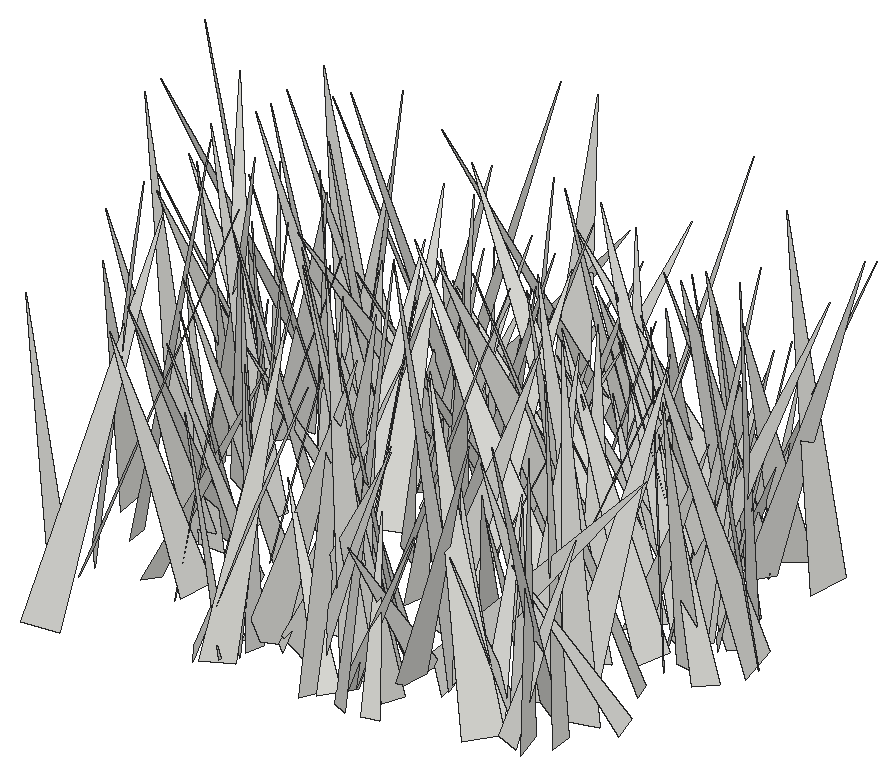
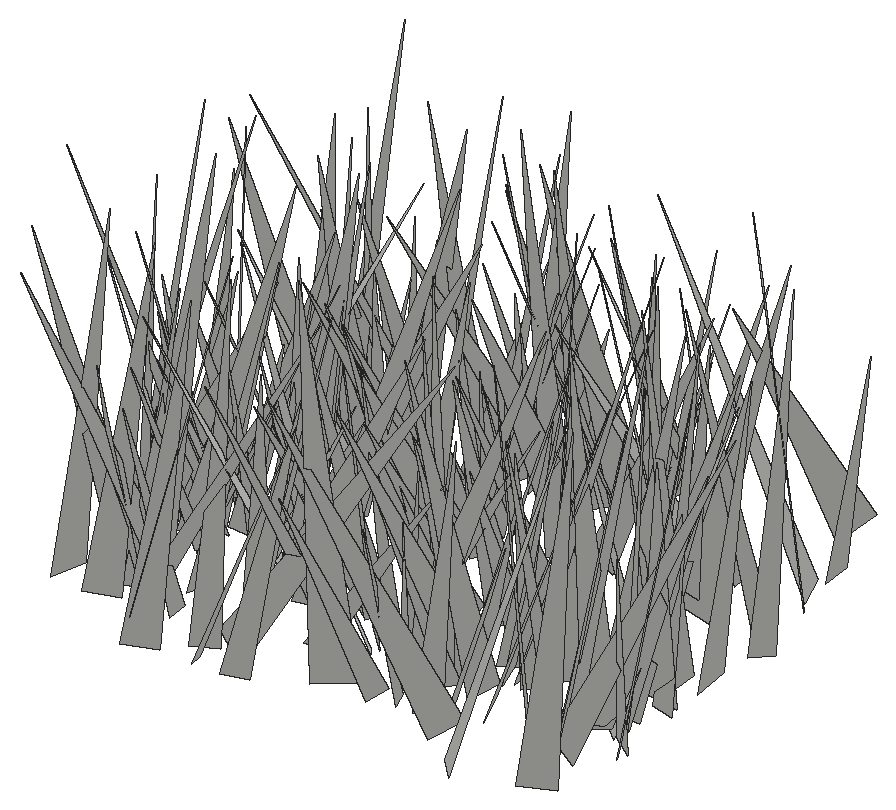
# SketchUp Ruby script. Lengths in inches.
U = 1.inch
M = Sketchup.active_model
def pt(a) = Geom::Point3d.new(a.map { |v| v * U })
def face(e, loops, mat)
  f = e.add_face(loops[0].map { |a| pt(a) })
  loops[1..].each { |l| e.add_face(l.map { |a| pt(a) }).erase! }
  f.material = f.back_material = mat if mat
  f
end
# faces: each face lists its corners as indices into pts; further lists are holes
def faces(e, pts, list, mat = nil) = list.each { |f| face(e, (f[0].is_a?(Array) ? f : [f]).map { |l| l.map { |i| pts[i] } }, mat) }
# xy, xz, yz: faces in a plane at the given z, y or x. An outline is a flat list of corners, or four numbers for a rectangle; further outlines are holes
def ring(l) = l.size == 4 ? [[l[0], l[1]], [l[2], l[1]], [l[2], l[3]], [l[0], l[3]]] : l.each_slice(2).to_a
def flat(e, list, mat, &to3) = list.each { |f| face(e, (f[0].is_a?(Array) ? f : [f]).map { |l| ring(l).map { |u, v| to3.(u, v) } }, mat) }
def xy(e, z, list, mat = nil) = flat(e, list, mat) { |x, y| [x, y, z] }
def xz(e, y, list, mat = nil) = flat(e, list, mat) { |x, z| [x, y, z] }
def yz(e, x, list, mat = nil) = flat(e, list, mat) { |y, z| [x, y, z] }
def lines(e, pts, list) = list.each { |a, b| e.add_line(pt(pts[a]), pt(pts[b])) }
# prism: a flat outline (further loops are holes) pulled along v
def prism(e, loops, v, mat = nil)
  f = face(e, loops, mat); d = Geom::Vector3d.new(v.map { |x| x * U })
  f.pushpull(f.normal.samedirection?(d) ? d.length : -d.length)
end
def box(e, o, s, mat = nil) = prism(e, [[o, [o[0] + s[0], o[1], o[2]], [o[0] + s[0], o[1] + s[1], o[2]], [o[0], o[1] + s[1], o[2]]]], [0, 0, s[2]], mat)
def at(x, y, z, deg = 0) = Geom::Transformation.translation(pt([x, y, z])) * Geom::Transformation.rotation(ORIGIN, Z_AXIS, deg.degrees)
def axes(o, x, y, z) = Geom::Transformation.new([*x, 0, *y, 0, *z, 0, *pt(o).to_a, 1])
def part(name) = M.definitions.add(name)
# library, detail: a bought-in or finely detailed component or shape, given as its bounding box
def library(name, o, s) = part(name).tap { |d| box(d.entities, o, s) }
def detail(e, o, s) = box(e.add_group.entities, o, s)
def put(e, d, t, mat = nil) = e.add_instance(d, t).tap { |i| i.material = mat if mat }
def group(e, t, mat = nil) = e.add_group.tap { |g| g.transformation = t; g.material = mat if mat }.entities
root = M.entities
c1 = part("fur_instance\#9")
p = [[0.8125,0,1.79],[0.67,-0.02,1.48],[0,-0.11,0],[0,0.11,0]]
faces(c1.entities,p,[[0,1,2,3]])
put(root,c1,axes([81.24,251.64,-27.1],[-0.33834,3.74046,0.53618],[3.75079,0.26714,0.50319],[-0.45836,-0.57497,3.72187]))
put(root,c1,axes([77.7,252.72,-27.1],[3.43659,4.37627,1.35344],[4.55407,-3.08156,-1.59944],[0.49399,-2.03617,5.32951]))
put(root,c1,axes([79.35,252.71,-27.1],[3.86855,-0.79855,0.19754],[-0.81455,-3.85123,0.38332],[-0.11496,0.41562,3.93147]))
put(root,c1,axes([73.47,251.37,-27.1],[4.56753,3.50086,0.36537],[3.49009,-4.58212,0.27435],[-0.45689,-0.00383,5.74831]))
put(root,c1,axes([78.98,252.12,-27.1],[-2.26305,3.25436,0.20739],[3.19812,2.16563,0.91504],[-0.63708,-0.68879,3.8568]))
put(root,c1,axes([74.48,251.8,-27.1],[-4.28089,-1.18354,0.47624],[-1.27514,3.91753,-1.72642],[-0.03977,1.79046,4.09221]))
put(root,c1,axes([86.23,255.7,-27.1],[-2.59583,-7.17613,0.91864],[-6.91744,2.74775,1.9178],[2.11891,0.17907,7.38629]))
put(root,c1,axes([66.48,252.56,-27.1],[-5.31115,0.249,1.00047],[0.14264,5.37711,-0.58108],[1.02108,0.54405,5.28514]))
put(root,c1,axes([76,253.87,-27.1],[0.54416,-5.67013,1.84078],[-5.27926,0.40028,2.79359],[2.76917,1.87733,4.9641]))
put(root,c1,axes([80.71,254.57,-27.1],[6.6655,-1.52718,0.22941],[-1.49066,-6.62814,-0.81212],[-0.40351,-0.74118,6.78982]))
put(root,c1,axes([80.7,255.67,-27.1],[3.27584,-2.78093,0.2499],[-2.38988,-2.99185,-1.96583],[-1.44378,-1.35736,3.82103]))
put(root,c1,axes([86.86,253.57,-27.1],[5.38301,1.51294,2.42188],[1.75431,-5.82988,-0.25732],[-2.2532,-0.92457,5.58566]))
put(root,c1,axes([74.49,251.45,-27.1],[-4.85985,3.92503,1.53679],[3.59209,5.08366,-1.6245],[2.20555,0.36911,6.032]))
put(root,c1,axes([85.26,253.01,-27.1],[-5.2406,4.407,1.34408],[4.57378,5.22157,0.71269],[0.55566,-1.41624,6.81011]))
put(root,c1,axes([78.59,251.73,-27.1],[-7.01527,0.64484,2.20419],[0.06996,7.14138,-1.86657],[2.29551,1.75305,6.79307]))
put(root,c1,axes([68.03,249.48,-27.1],[-6.65412,4.03174,0.74119],[3.28122,6.08544,-3.64454],[2.45722,2.79179,6.87384]))
put(root,c1,axes([74.87,253.57,-27.1],[5.22316,-4.20753,1.34718],[-4.41725,-5.01042,1.47756],[-0.07792,1.998,6.54228]))
put(root,c1,axes([79.34,253.47,-27.1],[-7.46216,1.5868,2.36089],[1.65538,7.81249,-0.01867],[2.31332,-0.47194,7.62898]))
put(root,c1,axes([70.68,255,-27.1],[-5.0365,1.95588,2.0654],[2.56555,4.93734,1.5806],[1.22852,-2.29236,5.16658]))
put(root,c1,axes([85.71,254.51,-27.1],[-3.47043,-1.20582,0.35373],[-1.16309,3.47557,0.43669],[0.47575,-0.29913,3.64791]))
put(root,c1,axes([70.1,254.63,-27.1],[4.41125,2.39111,1.26664],[2.67652,-4.21168,-1.37073],[-0.39751,-1.82353,4.82677]))
put(root,c1,axes([86.12,253.31,-27.1],[1.17442,4.10835,0.87727],[4.16659,-1.02282,-0.78793],[0.5364,-1.0501,4.19964]))
put(root,c1,axes([79.95,251.55,-27.1],[4.59054,6.55576,1.84003],[6.00661,-4.94402,2.62946],[-3.20693,0.124,7.5589]))
put(root,c1,axes([79.47,255.84,-27.1],[-3.91198,-5.41617,1.52932],[-5.50053,4.07361,0.35664],[1.19076,1.02376,6.67167]))
put(root,c1,axes([74.93,253,-27.1],[-6.75602,-0.97126,1.58692],[-1.43223,6.52998,-2.10085],[1.1876,2.34979,6.49412]))
put(root,c1,axes([85.06,253.69,-27.1],[-1.60634,4.05647,0.77587],[4.09581,1.67158,-0.25963],[0.53033,-0.623,4.35521]))
put(root,c1,axes([74.64,252.46,-27.1],[5.18637,5.57386,2.23152],[5.04396,-5.64447,2.37581],[-3.2567,0.13438,7.23339]))
put(root,c1,axes([81.04,253.19,-27.1],[-7.866,-1.33504,0.19154],[-1.32695,7.45779,-2.51268],[-0.24134,2.50839,7.5725]))
put(root,c1,axes([83.48,255.16,-27.1],[-3.08367,2.72536,1.78242],[3.08151,3.23588,0.38343],[1.05304,-1.48834,4.09751]))
put(root,c1,axes([72.75,255.79,-27.1],[-2.53313,-4.37285,1.78451],[-4.47538,2.86942,0.67851],[1.50904,1.16947,5.00781]))
put(root,c1,axes([66.24,254.74,-27.1],[5.70767,4.90783,2.44546],[5.23724,-5.92496,-0.33273],[-1.62433,-1.85811,7.52021]))
put(root,c1,axes([66.44,254.03,-27.1],[7.55875,3.30018,0.58934],[3.3113,-7.57673,-0.04195],[-0.52327,-0.27436,8.24768]))
put(root,c1,axes([81.13,255.56,-27.1],[5.03462,6.0848,0.40692],[5.07887,-3.8915,-4.64748],[3.37572,-3.22012,6.38538]))
put(root,c1,axes([85.7,254.42,-27.1],[-3.90689,0.46662,1.17538],[0.26281,4.03296,-0.72751],[1.23701,0.61693,3.86682]))
put(root,c1,axes([88.72,256.73,-27.1],[-4.09373,-0.36711,0.23804],[-0.24891,3.79616,1.57392],[0.35983,-1.55061,3.79686]))
put(root,c1,axes([75.23,253.98,-27.1],[3.93505,4.96293,0.50565],[4.97977,-3.8695,-0.7745],[0.29702,-0.87596,6.28613]))
put(root,c1,axes([72.21,256.62,-27.1],[-5.06877,-1.96642,0.89661],[-1.81084,5.11214,0.97466],[1.17965,-0.60192,5.34876]))
put(root,c1,axes([87.65,254.42,-27.1],[-6.31895,-1.30533,1.91515],[-1.71826,6.37081,-1.32708],[1.5554,1.73484,6.31441]))
put(root,c1,axes([81.94,255.74,-27.1],[-7.67624,-2.38765,2.18106],[-2.53698,7.93,-0.24775],[2.0054,0.89261,8.03519]))
put(root,c1,axes([70.76,257.75,-27.1],[-3.28751,-5.48957,1.02333],[-5.33666,3.43821,1.29963],[1.64396,0.18343,6.2653]))
put(root,c1,axes([68.89,254.69,-27.1],[4.92318,-0.35306,0.35659],[-0.43613,-4.74982,1.31852],[-0.24819,1.34315,4.75646]))
put(root,c1,axes([78.87,253.96,-27.1],[-4.6642,0.46344,0.8289],[0.1067,4.38406,-1.85075],[0.94364,1.79496,4.30631]))
put(root,c1,axes([69.5625,258.43,-27.1],[-1.29873,-6.18935,0.13887],[-6.18983,1.30082,0.08883],[0.11547,0.11765,6.32352]))
put(root,c1,axes([74.83,257.59,-27.1],[0.15208,-7.64456,1.76209],[-7.47072,0.39677,2.36609],[2.3943,1.72356,7.27077]))
put(root,c1,axes([84.03,257.16,-27.1],[-0.63245,-3.70623,0.66325],[-3.76509,0.62047,-0.12308],[-0.01169,0.67448,3.75779]))
put(root,c1,axes([79.77,254.94,-27.1],[-7.1733,-2.93015,0.73361],[-2.97558,6.52972,-3.01478],[-0.51951,3.05896,7.13815]))
put(root,c1,axes([68.76,257.85,-27.1],[-0.74223,-7.02206,1.66779],[-7.14663,0.48084,-1.156],[-1.00829,1.76103,6.96591]))
put(root,c1,axes([77.93,257.5625,-27.1],[-1.24841,-4.57565,0.91997],[-4.66472,1.19209,-0.401],[-0.15278,0.99186,4.72592]))
put(root,c1,axes([80.73,259.07,-27.1],[5.43533,-0.93824,0.08866],[-0.80913,-4.91198,-2.3767],[-0.48317,-2.32876,4.97739]))
put(root,c1,axes([64.89,258.76,-27.1],[6.40589,-1.32849,1.4611],[-0.83624,-6.31798,-2.07823],[-1.78897,-1.80373,6.20333]))
put(root,c1,axes([87.33,255.98,-27.1],[-0.74799,6.94474,2.29097],[7.27165,0.46217,0.97314],[-0.77532,-2.36525,6.91678]))
put(root,c1,axes([73.6,256.96,-27.1],[-0.2537,5.53184,2.90433],[5.7111,-0.97344,2.35297],[-2.53371,-2.74807,5.0129]))
put(root,c1,axes([79.5,252.89,-27.1],[6.78257,3.66457,1.14232],[2.83952,-6.35069,3.51329],[-2.58286,2.6414,6.86216]))
put(root,c1,axes([72.43,253.53,-27.1],[5.32818,4.49942,0.50618],[3.89144,-4.95023,3.04014],[-2.31467,2.03493,6.2763]))
put(root,c1,axes([70.41,256.99,-27.1],[4.87544,3.99495,1.42226],[4.19795,-4.85335,-0.75795],[-0.59966,-1.4959,6.2574]))
put(root,c1,axes([84.94,256.16,-27.1],[-5.03968,3.97301,2.20808],[3.85689,5.48236,-1.06156],[2.40517,-0.46656,6.329]))
put(root,c1,axes([69.17,257.73,-27.1],[-0.51846,-5.08764,2.15235],[-5.51728,0.36879,-0.45728],[-0.27624,2.18298,5.0935]))
put(root,c1,axes([86.57,256.31,-27.1],[-2.09917,6.50868,2.06271],[6.47308,2.58358,-1.56477],[2.17184,-1.40938,6.65739]))
put(root,c1,axes([74.07,258.76,-27.1],[-6.35383,-3.10693,1.06991],[-3.1587,6.41685,-0.12448],[0.9057,0.58302,7.07168]))
put(root,c1,axes([80.125,258.72,-27.1],[-0.83956,4.61048,2.28414],[5.1209,0.52371,0.82514],[-0.50027,-2.37653,4.61309]))
put(root,c1,axes([79.14,258.06,-27.1],[2.35297,-5.60644,2.50548],[-6.03434,-1.6135,2.05656],[1.13856,3.03489,5.72182]))
put(root,c1,axes([77.17,259.27,-27.1],[4.35751,-1.25814,0.68683],[-1.21703,-4.4086,-0.35441],[-0.75729,-0.15444,4.52164]))
put(root,c1,axes([82.36,259.78,-27.1],[-3.76395,0.54517,1.33918],[0.93594,3.7652,1.09781],[1.1021,-1.33566,3.64133]))
put(root,c1,axes([66.54,256.83,-27.1],[6.51752,3.06728,2.32468],[2.5593,-6.86862,1.88745],[-2.87443,0.8392,6.95153]))
put(root,c1,axes([71.23,258.59,-27.1],[3.50621,1.98379,0.78234],[2.0421,-3.55715,-0.13217],[-0.61424,-0.50223,4.02634]))
put(root,c1,axes([76.26,255.5,-27.1],[-5.16112,5.15909,0.10388],[4.87926,4.92701,-2.27629],[1.67923,1.54029,6.93338]))
put(root,c1,axes([73.25,261.65,-27.1],[-4.74866,-3.13825,0.27488],[-2.86364,4.50737,1.98925],[1.31291,-1.51952,5.33303]))
put(root,c1,axes([87.54,259.14,-27.1],[-7.14593,-4.06809,0.00282],[-3.91681,6.87864,-2.22635],[-1.09909,1.93614,7.91562]))
put(root,c1,axes([79.96,257.66,-27.1],[4.40688,2.08061,0.00975],[2.02682,-4.29803,1.08102],[-0.47012,0.97349,4.75194]))
put(root,c1,axes([67.52,261.62,-27.1],[-1.15928,-6.64992,1.1524],[-6.36185,1.46707,2.06591],[2.25307,0.72087,6.42631]))
put(root,c1,axes([84.09,260.01,-27.1],[-6.8866,-1.44069,2.04712],[-1.4724,7.17733,0.09795],[2.02444,0.3193,7.035]))
put(root,c1,axes([84.875,259.62,-27.1],[-1.73257,6.85044,2.42635],[7.20837,1.30251,1.46979],[-0.92468,-2.68187,6.91158]))
put(root,c1,axes([82.83,258.6875,-27.1],[5.42276,2.60915,0.23648],[2.58182,-5.41452,0.53583],[-0.44475,0.3811,5.9939]))
put(root,c1,axes([73,260.39,-27.1],[-5.77727,-4.35757,2.82703],[-4.73437,6.15702,-0.18467],[2.13687,1.8601,7.23403]))
put(root,c1,axes([74.89,261.64,-27.1],[-1.05562,-3.90874,0.84941],[-3.49411,1.32871,1.77194],[1.94702,0.26528,3.64044]))
put(root,c1,axes([83.32,259.98,-27.1],[-5.71693,5.39586,0.3581],[5.20349,5.34707,2.50186],[-1.47216,-2.05434,7.45247]))
put(root,c1,axes([87.9375,261.42,-27.1],[-0.39451,-5.89979,1.57703],[-6.09619,0.47415,0.24879],[0.36204,1.55494,5.90773]))
put(root,c1,axes([86.67,261.41,-27.1],[-4.90081,-4.60842,2.76686],[-4.75517,5.4628,0.67611],[2.50627,1.35324,6.69315]))
put(root,c1,axes([89.03,260.87,-27.1],[-2.03282,4.17049,1.29504],[4.34211,1.77825,1.08919],[-0.46493,-1.62705,4.50988]))
put(root,c1,axes([86.41,261.17,-27.1],[-6.01632,2.22797,0.81671],[2.32649,5.97644,0.83455],[0.46722,-1.07014,6.36109]))
put(root,c1,axes([68.51,260.35,-27.1],[-3.5127,-1.06556,1.8883],[-1.54789,3.74984,-0.76344],[1.51826,1.35772,3.59049]))
put(root,c1,axes([74.625,259.61,-27.1],[3.7445,3.22853,1.26331],[2.91821,-3.9391,1.41711],[-1.87174,0.31742,4.73672]))
put(root,c1,axes([69.54,260.64,-27.1],[-7.31689,1.04904,1.18508],[0.99417,7.40794,-0.41938],[1.23147,0.25252,7.3798]))
put(root,c1,axes([78.73,258.59,-27.1],[5.48783,2.36239,1.1528],[1.72376,-5.24883,2.55038],[-1.98455,1.97355,5.40302]))
put(root,c1,axes([89.56,263.18,-27.1],[-7.48109,-1.28394,1.71532],[-0.94889,7.57103,1.5286],[1.92105,-1.26035,7.43496]))
put(root,c1,axes([65.84,262.02,-27.1],[6.8953,0.9557,1.85973],[1.13553,-7.09282,-0.56526],[-1.75571,-0.83402,6.93822]))
put(root,c1,axes([65.09,261.39,-27.1],[-7.05246,-0.20222,1.59365],[-0.38202,7.18084,-0.77939],[1.56034,0.84409,7.01218]))
put(root,c1,axes([83.24,261.89,-27.1],[3.99343,-3.31881,2.86458],[-3.84361,-4.5142,0.12826],[-2.10878,1.94301,5.19091]))
put(root,c1,axes([79.55,265.81,-27.1],[6.1806,-4.85252,1.92283],[-3.89661,-6.27237,-3.30423],[-3.47285,-1.59827,7.12944]))
put(root,c1,axes([65.15,264.0625,-27.1],[-2.48382,-6.27006,1.58629],[-6.2632,2.75568,1.08533],[1.61318,1.04494,6.65621]))
put(root,c1,axes([78.77,259.98,-27.1],[-3.2571,5.60614,0.8435],[5.30317,3.35677,-1.83235],[2.00417,0.22864,6.21933]))
put(root,c1,axes([89.16,263.49,-27.1],[-5.20637,-5.83633,2.28098],[-6.06397,5.44004,0.07832],[1.57922,1.64775,7.82067]))
put(root,c1,axes([72.2,261.05,-27.1],[5.46763,0.70402,1.09334],[0.38726,-5.3924,1.5356],[-1.2414,1.41859,5.29457]))
put(root,c1,axes([66.1,265.23,-27.1],[2.22572,-6.24997,0.53761],[-6.03536,-2.28904,-1.62473],[-1.71046,-0.05581,6.43243]))
put(root,c1,axes([87.14,262.48,-27.1],[3.46953,-2.67132,1.40146],[-2.94376,-3.4648,0.68347],[-0.65905,1.41311,4.3251]))
put(root,c1,axes([84.59,262.52,-27.1],[3.70527,-2.55389,0.75103],[-2.66189,-3.54115,1.0909],[0.02774,1.32414,4.36593]))
put(root,c1,axes([66.91,263.76,-27.1],[4.97052,1.68586,2.30908],[2.28367,-5.12743,-1.17229],[-1.72012,-1.9358,5.11604]))
put(root,c1,axes([83.84,260.62,-27.1],[2.91229,5.1803,0.24137],[5.15397,-2.92189,0.52374],[-0.57474,0.04729,5.91968]))
put(root,c1,axes([82.65,264.82,-27.1],[5.01646,-0.03484,2.02413],[0.79085,-4.94522,-2.0451],[-1.86357,-2.19241,4.58078]))
put(root,c1,axes([78.0625,259.57,-27.1],[7.02675,2.35333,1.41841],[1.60681,-6.67867,3.12071],[-2.22895,2.60433,6.72121]))
put(root,c1,axes([70.99,261.76,-27.1],[0.97276,4.45119,0.9772],[4.35496,-1.20232,1.14148],[-1.3425,-0.67498,4.41093]))
put(root,c1,axes([69.21,264.5625,-27.1],[4.90376,-2.85552,0.72078],[-2.73926,-4.93651,-0.92072],[-1.08166,-0.44414,5.59939]))
put(root,c1,axes([74.5625,264.87,-27.1],[6.47505,-0.26988,1.20187],[0.07267,-6.33614,-1.81428],[-1.22965,-1.79557,6.22153]))
put(root,c1,axes([85.27,264.95,-27.1],[-5.50457,-1.9976,0.13924],[-1.94432,5.42927,1.02602],[0.47897,-0.91798,5.76524]))
put(root,c1,axes([84.88,263.25,-27.1],[0.57769,-3.84784,2.16026],[-4.16363,-1.197,-1.01866],[-1.46176,1.88882,3.75525]))
put(root,c1,axes([86.97,263.22,-27.1],[3.29573,-2.04708,1.27302],[-2.29025,-3.33183,0.57152],[-0.75223,1.17531,3.83742]))
put(root,c1,axes([71.38,264.89,-27.1],[3.60801,-2.69307,1.35493],[-2.4926,-3.85347,-1.02171],[-1.69571,-0.06573,4.3848]))
put(root,c1,axes([80.42,263.92,-27.1],[6.04949,2.12455,0.78775],[2.22415,-5.99674,-0.90711],[-0.43293,-1.1207,6.34722]))
put(root,c1,axes([88.34,263.71,-27.1],[-1.48445,-5.73193,2.26963],[-5.6541,0.33538,-2.85107],[-2.45713,2.69116,5.18942]))
put(root,c1,axes([65.57,266.43,-27.1],[-4.43936,-4.76816,0.23664],[-4.66276,4.39992,1.18262],[1.02469,-0.63608,6.40661]))
put(root,c1,axes([80.88,264.01,-27.1],[4.18181,1.0835,0.53294],[1.13424,-4.18373,-0.39425],[-0.41412,-0.51766,4.30187]))
put(root,c1,axes([70.5,265.05,-27.1],[-7.46338,-1.41905,1.28497],[-1.31215,7.55774,0.72509],[1.39396,-0.48353,7.56241]))
put(root,c1,axes([86.04,264.04,-27.1],[-6.89397,4.20656,1.53795],[4.42912,6.82252,1.19307],[0.66584,-1.82904,7.9874]))
put(root,c1,axes([84.45,265.8,-27.1],[-3.67064,-4.64361,1.03864],[-4.58105,3.8034,0.81465],[1.28682,0.29416,5.86285]))
put(root,c1,axes([70.83,269.07,-27.1],[-6.33754,-5.19611,0.8236],[-4.02771,5.62162,4.47406],[3.3846,-3.03975,6.86635]))
put(root,c1,axes([88.79,263.92,-27.1],[-6.27895,-2.5321,2.5957],[-2.9165,6.61067,-0.60625],[2.15482,1.56906,6.74309]))
put(root,c1,axes([67.01,267.01,-27.1],[-3.15588,-6.30761,0.73503],[-6.08642,3.23856,1.65924],[1.81157,-0.10755,6.85511]))
put(root,c1,axes([77.24,264.9375,-27.1],[3.19208,-3.97574,0.46961],[-3.91795,-2.97897,1.41133],[0.82265,1.2392,4.89939]))
put(root,c1,axes([85.54,263.65,-27.1],[3.97232,6.71602,1.21655],[6.692,-3.55551,-2.22255],[1.34242,-2.14887,7.47961]))
put(root,c1,axes([72.18,263.24,-27.1],[-2.71251,3.20119,0.88639],[3.03008,2.85354,-1.03292],[1.36084,0.02704,4.06674]))
put(root,c1,axes([66.04,266.39,-27.1],[2.61473,-6.42495,0.46001],[-6.33227,-2.47287,1.45453],[1.18065,0.96609,6.78241]))
put(root,c1,axes([86.2,262.27,-27.1],[3.78632,3.0497,0.88341],[2.42458,-3.66486,2.25998],[-2.05,1.29824,4.30457]))
put(root,c1,axes([73.32,262.62,-27.1],[-3.56616,5.34471,0.77163],[5.27091,3.64619,-0.89538],[1.17426,-0.13507,6.36253]))
put(root,c1,axes([82.24,265.49,-27.1],[-2.77092,-3.22119,0.17285],[-3.17409,2.68192,-0.90354],[-0.57541,0.71776,4.15182]))
put(root,c1,axes([86.47,262.51,-27.1],[3.93079,5.90323,1.06815],[5.73682,-4.07234,1.39466],[-1.7544,-0.09002,6.95371]))
put(root,c1,axes([87.5,263.45,-27.1],[-3.93965,-2.75758,3.63418],[-3.8658,4.56754,-0.72493],[2.42222,2.80458,4.7539]))
put(root,c1,axes([75.03,264.77,-27.1],[6.15775,0.09619,0.89999],[0.03195,-6.20791,0.44493],[-0.90455,0.43558,6.14241]))
put(root,c1,axes([65.3,265.94,-27.1],[-2.6203,-2.567,1.06702],[-2.53846,2.80716,0.51965],[1.13325,0.35259,3.63117]))
put(root,c1,axes([80.96,265.7,-27.1],[-0.62514,-3.66803,1.11265],[-3.82799,0.53943,-0.37244],[-0.19721,1.15663,3.70223]))
put(root,c1,axes([74.94,266.88,-27.1],[-1.76635,-5.02439,0.02248],[-4.81779,1.68692,-1.51928],[-1.42615,0.52421,5.10454]))
put(root,c1,axes([71.01,265.39,-27.1],[-6.09908,-2.25868,1.59557],[-2.41433,6.23322,-0.4051],[1.3485,0.94419,6.49124]))
put(root,c1,axes([65.8,266.12,-27.1],[-4.26864,3.3889,1.68719],[3.78174,3.93314,1.66776],[0.17248,-2.36607,5.18889]))
put(root,c1,axes([69.72,265.5625,-27.1],[2.82184,-3.33686,1.43593],[-3.57868,-2.86589,0.37288],[-0.62414,1.34588,4.35412]))
put(root,c1,axes([65.79,263.49,-27.1],[-1.06159,6.87885,0.56166],[6.76624,0.92524,1.45707],[-1.36093,-0.76575,6.80607]))
put(root,c1,axes([82.52,265.01,-27.1],[0.52075,4.40411,1.27547],[4.58416,-0.47433,-0.2338],[0.09203,-1.29345,4.42863]))
put(root,c1,axes([84.99,268.5,-27.1],[5.51708,-5.76072,0.82028],[-5.55442,-5.55067,-1.6234],[-1.73412,-0.54876,7.80952]))
put(root,c1,axes([74.58,262.94,-27.1],[5.42,0.95377,1.93695],[-0.10115,-5.11614,2.80228],[-2.15667,2.63692,4.73638]))
put(root,c1,axes([83.53,267.43,-27.1],[-6.08575,-1.31512,1.93305],[-0.80976,6.24223,1.69745],[2.19329,-1.34444,5.99037]))
put(root,c1,axes([73.6875,264.57,-27.1],[-0.65991,4.20046,0.70673],[4.09857,0.8209,-1.05196],[1.15975,-0.51096,4.1198]))
put(root,c1,axes([73.64,265.79,-27.1],[-2.04646,-5.42862,2.85461],[-5.95901,2.47232,0.42963],[1.45222,2.49488,5.78561]))
put(root,c1,axes([72.125,265.98,-27.1],[-3.54918,2.04608,0.76374],[2.14815,3.53344,0.51649],[0.39398,-0.83357,4.06404]))
put(root,c1,axes([80.89,265.59,-27.1],[-4.85114,5.94494,0.47809],[5.69058,4.42924,2.66526],[-1.78556,-2.03568,7.19529]))
put(root,c1,axes([74.8125,266.99,-27.1],[5.2345,0.58731,0.96902],[0.7581,-5.21929,-0.93179],[-0.84215,-1.04786,5.18428]))
put(root,c1,axes([87.11,266.1,-27.1],[-3.42512,-4.29344,1.99666],[-4.721,3.28594,-1.03273],[0.36395,2.21827,5.39431]))
put(root,c1,axes([74.28,267.02,-27.1],[1.30343,6.50873,4.51627],[7.0846,-3.00591,2.28737],[-3.54523,-3.61388,6.23141]))
put(root,c1,axes([74.25,267.03,-27.1],[-3.40135,-0.48301,1.73948],[-0.24917,3.80046,0.56808],[1.78802,-0.38922,3.38818]))
put(root,c1,axes([72.37,266.05,-27.1],[4.7492,-0.22527,1.39473],[-0.44396,-4.88167,0.72329],[-1.34124,0.81823,4.6992]))
put(root,c1,axes([84.89,265.34,-27.1],[0.96438,4.41888,0.40988],[4.43511,-0.94495,-0.24768],[0.15571,-0.45288,4.5161]))
put(root,c1,axes([64.78,266.92,-27.1],[-6.58446,-3.61184,1.85584],[-3.84727,6.67992,-0.64953],[1.29924,1.4758,7.48189]))
put(root,c1,axes([66.12,268.53,-27.1],[-2.71774,-6.73125,0.47193],[-6.54696,2.5072,-1.9416],[-1.63394,1.15011,6.99472]))
put(root,c1,axes([78.18,264.24,-27.1],[5.42222,1.22065,1.50489],[0.3801,-5.05507,2.73075],[-1.90005,2.47215,4.84081]))
put(root,c1,axes([75.9,267.125,-27.1],[3.62695,2.69385,0.06353],[2.59465,-3.4627,-1.30122],[0.7271,-1.08099,4.32648]))
put(root,c1,axes([69.95,267.81,-27.1],[-6.57116,-2.81105,0.67584],[-2.85659,6.57143,-0.44162],[0.44572,0.67315,7.13352]))
put(root,c1,axes([70.97,266.875,-27.1],[6.40804,-1.16691,1.44574],[-1.35043,-6.49108,0.74636],[-1.27601,1.00946,6.47052]))
put(root,c1,axes([66.57,268.12,-27.1],[-5.55068,-3.03255,1.58004],[-3.06213,5.7489,0.27653],[1.52193,0.50669,6.31901]))
put(root,c1,axes([67.4375,267.24,-27.1],[1.6675,5.06938,1.93589],[5.41393,-1.41673,-0.95346],[0.36831,-2.12629,5.25072]))
put(root,c1,axes([76.36,266.22,-27.1],[3.82909,4.88275,1.88302],[4.81565,-4.20088,1.10051],[-2.04855,-0.74856,6.10673]))
put(root,c1,axes([77.625,268.04,-27.1],[-3.75948,2.94392,0.27379],[2.73653,3.29698,2.12525],[-1.1194,-1.82718,4.27594]))
put(root,c1,axes([85.93,269.83,-27.1],[3.11864,-5.68803,0.55795],[-5.6529,-3.16353,-0.65398],[-0.84244,0.17118,6.45383]))
put(root,c1,axes([72.13,267.27,-27.1],[0.15011,3.96157,1.30257],[3.86973,0.35348,-1.52101],[1.55431,-1.26265,3.66102]))
put(root,c1,axes([64.6875,266.91,-27.1],[1.72426,4.07776,1.35625],[4.04188,-2.03524,0.98061],[-1.4597,-0.81871,4.31736]))
put(root,c1,axes([84.28,270.15,-27.1],[-5.52668,-3.91053,1.22579],[-3.5737,5.60606,1.77193],[2.00587,-0.78663,6.53427]))
put(root,c1,axes([80.7,270.53,-27.1],[0.16634,-6.6201,0.01552],[-6.42128,-0.15757,1.61124],[1.61035,0.05552,6.42319]))
put(root,c1,axes([71.54,269.35,-27.1],[3.51488,-3.51732,0.75482],[-3.443,-3.59499,-0.71937],[-1.04262,0.01399,4.9202]))
put(root,c1,axes([84.29,269.65,-27.1],[-7.00038,0.48524,0.02911],[0.47648,6.76613,1.79834],[-0.09628,-1.796,6.78283]))
put(root,c1,axes([79.54,269.33,-27.1],[-6.2182,-2.45212,1.53392],[-2.39925,6.40419,0.51167],[1.61537,0.0727,6.66461]))
put(root,c1,axes([81.72,264.54,-27.1],[5.15692,6.28398,0.1894],[5.87834,-4.90651,2.73667],[-2.22922,1.59869,7.6546]))
put(root,c1,axes([85.41,268.58,-27.1],[1.48907,3.83094,1.46531],[4.09712,-1.31638,-0.722],[0.19182,-1.62223,4.04625]))
put(root,c1,axes([74.06,267.43,-27.1],[1.76698,3.75792,1.11012],[3.4505,-2.06932,1.51278],[-1.85698,-0.26926,3.86726]))
put(root,c1,axes([80.43,267.91,-27.1],[-5.1029,2.41175,1.4356],[2.37658,5.2976,-0.4521],[1.4931,-0.1897,5.62599]))
put(root,c1,axes([85.68,268.0625,-27.1],[6.84778,-1.68967,1.39359],[-1.92956,-6.81846,1.21431],[-1.03628,1.53061,6.94784]))
put(root,c1,axes([66.49,269.8,-27.1],[5.45903,4.38742,2.52703],[5.0114,-5.21201,-1.77686],[-0.72192,-3.00365,6.77446]))
put(root,c1,axes([79.92,270.04,-27.1],[-3.41379,-7.32141,0.63154],[-6.65452,2.7845,-3.69049],[-3.11756,2.07349,7.18591]))
put(root,c1,axes([87.94,269.1875,-27.1],[-7.15931,0.95304,2.49675],[1.12982,7.54938,0.35801],[2.42189,-0.70454,7.21359]))
put(root,c1,axes([84.82,267.39,-27.1],[6.67299,1.88656,0.54903],[1.75109,-6.59185,1.3677],[-0.89119,1.17381,6.79833]))
put(root,c1,axes([72.63,265.64,-27.1],[-6.96158,0.42843,3.50828],[-1.43896,6.73486,-3.67782],[3.22816,3.92599,5.92628]))
put(root,c1,axes([83.04,269.15,-27.1],[4.10361,0.18993,0.89205],[0.09258,-4.17709,0.46346],[-0.90734,0.43277,4.08178]))
put(root,c1,axes([78.53,271.53,-27.1],[3.73723,-3.51523,0.8829],[-3.22394,-3.80362,-1.49732],[-1.65607,-0.52811,4.90732]))
put(root,c1,axes([76.29,267.96,-27.1],[1.18506,6.07091,0.5983],[5.8889,-0.9794,-1.72625],[1.5921,-0.89616,5.93973]))
put(root,c1,axes([75.49,269.68,-27.1],[-3.47226,6.33449,3.63746],[6.89094,4.17667,-0.69553],[2.42317,-2.80055,7.19017]))
put(root,c1,axes([72.92,269.24,-27.1],[3.22488,1.438,0.95498],[1.40641,-3.36208,0.31327],[-1.00092,-0.09099,3.51704]))
put(root,c1,axes([82.5,271.95,-27.1],[3.11347,-5.57932,0.56956],[-5.54553,-3.1599,-0.63956],[-0.83685,0.18197,6.35716]))
put(root,c1,axes([80.36,271.47,-27.1],[-4.41173,-1.92667,0.46008],[-1.77307,4.34177,1.17998],[0.88316,-0.90777,4.66723]))
put(root,c1,axes([70.28,269.86,-27.1],[4.62991,-4.98565,0.093],[-4.3743,-3.99984,3.34189],[2.39393,2.33366,5.92659]))
put(root,c1,axes([65.17,271.14,-27.1],[3.62749,-5.55241,1.8821],[-5.65778,-3.89547,-0.58748],[-1.5366,1.23544,6.60627]))
put(root,c1,axes([68.53,272.04,-27.1],[-4.85913,-4.7221,0.69622],[-4.68141,4.90862,0.61965],[0.93132,0.03646,6.74725]))
put(root,c1,axes([73.76,269.43,-27.1],[3.57113,-2.0967,0.79041],[-2.23153,-3.1932,1.61171],[0.20288,1.78359,3.81464]))
